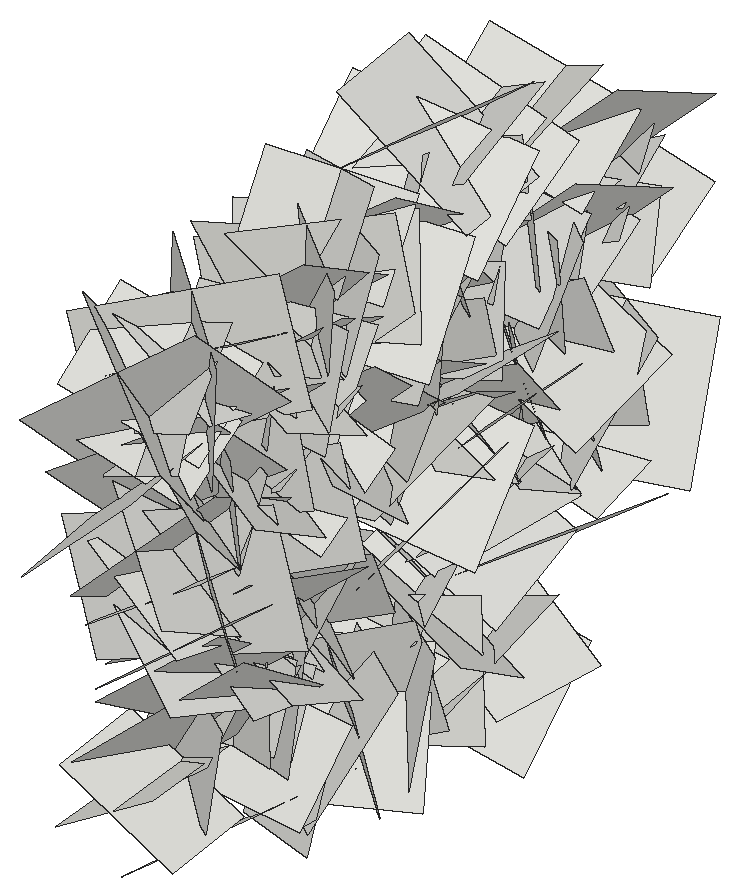
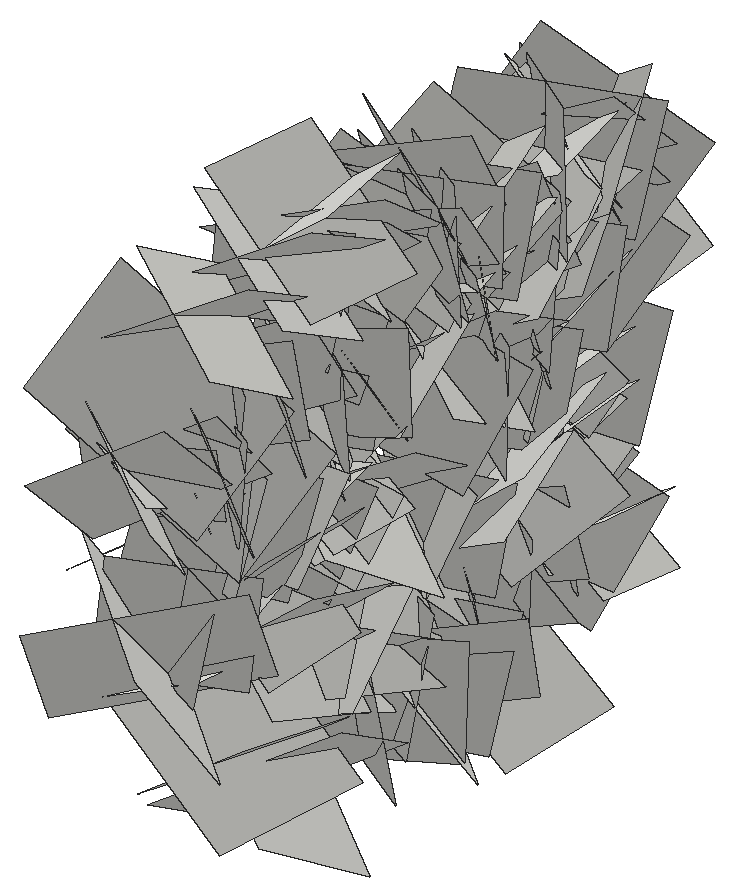
# SketchUp Ruby script. Lengths in inches.
U = 1.inch
M = Sketchup.active_model
def pt(a) = Geom::Point3d.new(a.map { |v| v * U })
def face(e, loops, mat)
  f = e.add_face(loops[0].map { |a| pt(a) })
  loops[1..].each { |l| e.add_face(l.map { |a| pt(a) }).erase! }
  f.material = f.back_material = mat if mat
  f
end
# faces: each face lists its corners as indices into pts; further lists are holes
def faces(e, pts, list, mat = nil) = list.each { |f| face(e, (f[0].is_a?(Array) ? f : [f]).map { |l| l.map { |i| pts[i] } }, mat) }
# xy, xz, yz: faces in a plane at the given z, y or x. An outline is a flat list of corners, or four numbers for a rectangle; further outlines are holes
def ring(l) = l.size == 4 ? [[l[0], l[1]], [l[2], l[1]], [l[2], l[3]], [l[0], l[3]]] : l.each_slice(2).to_a
def flat(e, list, mat, &to3) = list.each { |f| face(e, (f[0].is_a?(Array) ? f : [f]).map { |l| ring(l).map { |u, v| to3.(u, v) } }, mat) }
def xy(e, z, list, mat = nil) = flat(e, list, mat) { |x, y| [x, y, z] }
def xz(e, y, list, mat = nil) = flat(e, list, mat) { |x, z| [x, y, z] }
def yz(e, x, list, mat = nil) = flat(e, list, mat) { |y, z| [x, y, z] }
def lines(e, pts, list) = list.each { |a, b| e.add_line(pt(pts[a]), pt(pts[b])) }
# prism: a flat outline (further loops are holes) pulled along v
def prism(e, loops, v, mat = nil)
  f = face(e, loops, mat); d = Geom::Vector3d.new(v.map { |x| x * U })
  f.pushpull(f.normal.samedirection?(d) ? d.length : -d.length)
end
def box(e, o, s, mat = nil) = prism(e, [[o, [o[0] + s[0], o[1], o[2]], [o[0] + s[0], o[1] + s[1], o[2]], [o[0], o[1] + s[1], o[2]]]], [0, 0, s[2]], mat)
def at(x, y, z, deg = 0) = Geom::Transformation.translation(pt([x, y, z])) * Geom::Transformation.rotation(ORIGIN, Z_AXIS, deg.degrees)
def axes(o, x, y, z) = Geom::Transformation.new([*x, 0, *y, 0, *z, 0, *pt(o).to_a, 1])
def part(name) = M.definitions.add(name)
# library, detail: a bought-in or finely detailed component or shape, given as its bounding box
def library(name, o, s) = part(name).tap { |d| box(d.entities, o, s) }
def detail(e, o, s) = box(e.add_group.entities, o, s)
def put(e, d, t, mat = nil) = e.add_instance(d, t).tap { |i| i.material = mat if mat }
def group(e, t, mat = nil) = e.add_group.tap { |g| g.transformation = t; g.material = mat if mat }.entities
root = M.entities
c1 = part("Component\#6")
p = [[0.01,0,0],[0,3.24,4.54],[4.32,3.24,4.54],[4.33,0,0]]
faces(c1.entities,p,[[0,1,2,3]])
put(root,c1,axes([400.91,192.58,32.17],[0.11188,-0.86522,-0.03173],[-0.14554,-0.04829,0.85998],[0.90613,0.09907,0.14204]))
put(root,c1,axes([400.91,194.3125,23.26],[-0.02367,-0.75059,-0.08188],[0.02978,-0.08269,0.75031],[0.79979,-0.01914,-0.03036]))
put(root,c1,axes([404.88,194.3125,23.26],[0.02367,-0.75059,-0.08188],[-0.02978,-0.08269,0.75031],[-0.79979,-0.01914,-0.03036]))
put(root,c1,axes([400.91,192.15,39.48],[-0.21361,0.71392,-0.72381],[-0.12034,-0.74908,-0.70723],[1.07091,0.05823,-0.22384]))
put(root,c1,axes([404.88,192.15,39.48],[0.21361,0.71392,-0.72381],[0.12034,-0.74908,-0.70723],[-1.07091,0.05823,-0.22384]))
put(root,c1,axes([404.88,191.375,35.34],[-0.1473,0.40574,0.51918],[-0.07991,0.51733,-0.42447],[-0.69387,-0.14571,-0.06134]))
put(root,c1,axes([400.91,191.375,35.34],[0.1473,0.40574,0.51918],[0.07991,0.51733,-0.42447],[0.69387,-0.14571,-0.06134]))
put(root,c1,axes([404.88,195.16,37.28],[-0.08536,-0.54597,-0.55526],[-0.06407,-0.55215,0.55168],[-0.82294,0.09962,0.01464]))
put(root,c1,axes([400.91,195.16,37.28],[0.08536,-0.54597,-0.55526],[0.06407,-0.55215,0.55168],[0.82294,0.09962,0.01464]))
put(root,c1,axes([400.91,194.17,31.15],[-0.1572,-0.65225,0.62778],[-0.00257,0.63643,0.66066],[0.9596,-0.10514,0.10461]))
put(root,c1,axes([404.88,194.17,31.15],[0.1572,-0.65225,0.62778],[0.00257,0.63643,0.66066],[-0.9596,-0.10514,0.10461]))
put(root,c1,axes([400.91,192.38,31.46],[0.05244,0.73173,-0.11131],[0.01157,-0.11227,-0.73318],[0.78447,-0.04726,0.01825]))
put(root,c1,axes([404.88,192.38,31.46],[-0.05244,0.73173,-0.11131],[-0.01157,-0.11227,-0.73318],[-0.78447,-0.04726,0.01825]))
put(root,c1,axes([400.91,192.76,27.5],[-0.21382,-0.08753,1.03604],[0.20559,1.03367,0.1251],[1.08277,-0.21355,0.18084]))
put(root,c1,axes([400.91,193.07,33.95],[0.05953,0.85388,-0.40475],[-0.24794,-0.38029,-0.83472],[0.97048,-0.14953,-0.18843]))
put(root,c1,axes([404.88,193.07,33.95],[-0.05953,0.85388,-0.40475],[0.24794,-0.38029,-0.83472],[-0.97048,-0.14953,-0.18843]))
put(root,c1,axes([404.88,192.62,23.41],[0.0945,0.05137,0.75973],[-0.00531,0.76494,-0.05113],[-0.80713,0.00098,0.08928]))
put(root,c1,axes([404.88,193.25,29.42],[0.0602,0.67546,-0.3863],[0.10598,-0.39045,-0.66802],[-0.81797,-0.00088,-0.11498]))
put(root,c1,axes([400.91,194.92,22.54],[0.07164,-0.895,0.57486],[-0.24411,0.55005,0.88344],[1.1008,0.18023,0.15849]))
put(root,c1,axes([404.88,192.68,25.51],[-0.10584,0.56729,0.32604],[0.07365,0.33715,-0.56532],[-0.68964,-0.05105,-0.11041]))
put(root,c1,axes([404.88,195.4,26.27],[-0.15303,-0.80886,0.21466],[0.08059,0.20425,0.82078],[-0.8834,0.15875,0.0377]))
put(root,c1,axes([400.91,195.4,26.27],[0.15303,-0.80886,0.21466],[-0.08059,0.20425,0.82078],[0.8834,0.15875,0.0377]))
put(root,c1,axes([400.91,192.92,34.17],[-0.15147,-0.1521,1.01718],[-0.1212,1.02293,0.1369],[1.08344,0.09316,0.15752]))
put(root,c1,axes([404.88,192.92,34.17],[0.15147,-0.1521,1.01718],[0.1212,1.02293,0.1369],[-1.08344,0.09316,0.15752]))
put(root,c1,axes([400.91,195.89,35.57],[-0.03273,-0.74668,0.19464],[0.06894,0.19158,0.74527],[0.81502,-0.04619,-0.05522]))
put(root,c1,axes([404.88,195.89,35.57],[0.03273,-0.74668,0.19464],[-0.06894,0.19158,0.74527],[-0.81502,-0.04619,-0.05522]))
put(root,c1,axes([404.88,194.0625,27.88],[0.03826,-0.32146,0.75655],[0.14724,0.74878,0.31153],[-0.85881,0.11405,0.08712]))
put(root,c1,axes([404.88,194.18,31.13],[0.04063,-0.16003,0.87853],[0.02386,0.87924,0.15917],[-0.94627,0.0153,0.04174]))
put(root,c1,axes([400.91,194.18,31.13],[-0.04063,-0.16003,0.87853],[-0.02386,0.87924,0.15917],[0.94627,0.0153,0.04174]))
put(root,c1,axes([404.88,194.1,30.97],[0.07757,0.18705,0.69229],[-0.05179,0.69557,-0.18277],[-0.75837,-0.02837,0.08329]))
put(root,c1,axes([400.91,194.12,36.42],[-0.16155,0.92195,-0.51802],[0.06641,-0.51458,-0.93426],[1.119,0.16364,-0.01934]))
put(root,c1,axes([404.88,194.71,36.49],[0.01491,0.71707,-0.22931],[0.11795,-0.22881,-0.70868],[-0.78925,-0.02064,-0.11024]))
put(root,c1,axes([404.88,197.53,26.62],[-0.11622,-0.11144,-0.6986],[-0.08861,-0.69994,0.12478],[-0.74462,0.10068,0.09418]))
put(root,c1,axes([400.91,197.53,26.62],[0.11622,-0.11144,-0.6986],[0.08861,-0.69994,0.12478],[0.74462,0.10068,0.09418]))
put(root,c1,axes([404.88,198.41,25.5],[0.14641,-1.02966,0.26735],[0.10928,0.28128,1.03005],[-1.12233,-0.10694,0.13517]))
put(root,c1,axes([400.91,198.41,25.5],[-0.14641,-1.02966,0.26735],[-0.10928,0.28128,1.03005],[1.12233,-0.10694,0.13517]))
put(root,c1,axes([400.91,198.72,19.65],[-0.06387,-1.04135,0.05905],[-0.06023,0.06234,1.04135],[1.10396,-0.05685,0.06023]))
put(root,c1,axes([400.91,195.45,23.05],[0.08121,0.42866,0.62692],[0.16296,0.6083,-0.43472],[0.78836,-0.1699,0.02528]))
put(root,c1,axes([400.91,198.57,33.25],[-0.09717,0.14422,-0.89801],[-0.11089,-0.89824,-0.13357],[0.95769,-0.08937,-0.10658]))
put(root,c1,axes([404.88,198.57,33.25],[0.09717,0.14422,-0.89801],[0.11089,-0.89824,-0.13357],[-0.95769,-0.08937,-0.10658]))
put(root,c1,axes([400.91,195.7,29.31],[-0.12944,0.87645,-0.3909],[0.13192,-0.37627,-0.88251],[1.00866,0.16168,0.06525]))
put(root,c1,axes([400.91,196.41,37.05],[0.02372,0.78814,-0.36288],[0.15491,-0.36124,-0.77556],[0.90659,0.0411,0.14202]))
put(root,c1,axes([404.88,195.33,34.42],[-0.12228,0.30682,0.85432],[0.19875,0.85067,-0.2802],[-0.94146,0.13973,-0.17012]))
put(root,c1,axes([400.91,195.33,34.42],[0.12228,0.30682,0.85432],[-0.19875,0.85067,-0.2802],[0.94146,0.13973,-0.17012]))
put(root,c1,axes([400.91,200.17,25.9],[0.12286,-0.34825,-0.84521],[-0.12526,-0.85054,0.33424],[0.96086,-0.06635,0.15165]))
put(root,c1,axes([400.91,196.95,39.61],[-0.06663,0.78722,-0.39485],[-0.0883,-0.3994,-0.78302],[0.92935,0.01849,-0.10271]))
put(root,c1,axes([404.88,196.95,39.61],[0.06663,0.78722,-0.39485],[0.0883,-0.3994,-0.78302],[-0.92935,0.01849,-0.10271]))
put(root,c1,axes([404.88,199.74,34.07],[-0.11183,-0.60219,-0.2199],[0.02555,-0.22643,0.6085],[-0.67907,0.09065,0.0591]))
put(root,c1,axes([404.88,197.11,20.7],[0.0234,0.20043,0.60552],[-0.11848,0.59772,-0.19378],[-0.66563,-0.09934,0.05578]))
put(root,c1,axes([404.88,201.02,32],[0.03236,-0.79816,-0.43551],[0.07074,-0.43262,0.79753],[-0.9612,-0.0587,0.04403]))
put(root,c1,axes([400.91,201.02,32],[-0.03236,-0.79816,-0.43551],[-0.07074,-0.43262,0.79753],[0.9612,-0.0587,0.04403]))
put(root,c1,axes([400.91,200.08,36.17],[0.04967,-0.3024,-0.77978],[0.15753,-0.76557,0.30582],[0.87244,0.15545,-0.01082]))
put(root,c1,axes([404.88,196.5,26.6],[0.00001,0.64808,0.59207],[0.20568,0.57742,-0.63205],[-0.90746,0.13088,-0.14325]))
put(root,c1,axes([404.88,198.68,37.125],[-0.06347,0.58127,-0.24952],[0.07215,-0.24326,-0.58302],[-0.66662,-0.08167,-0.03935]))
put(root,c1,axes([400.91,201.02,39.48],[-0.13577,0.09163,-0.9618],[-0.05798,-0.96935,-0.08506],[1.02248,-0.0428,-0.13253]))
put(root,c1,axes([404.88,201.02,39.48],[0.13577,0.09163,-0.9618],[0.05798,-0.96935,-0.08506],[-1.02248,-0.0428,-0.13253]))
put(root,c1,axes([404.88,199.18,25.47],[-0.11604,-0.3767,0.6399],[0.02749,0.64448,0.38383],[-0.78661,0.07809,-0.08099]))
put(root,c1,axes([400.91,199.18,25.47],[0.11604,-0.3767,0.6399],[-0.02749,0.64448,0.38383],[0.78661,0.07809,-0.08099]))
put(root,c1,axes([400.91,197.17,21.41],[-0.31691,0.51794,0.91951],[-0.05422,0.94746,-0.55031],[1.11735,0.19287,0.23409]))
put(root,c1,axes([404.88,197.17,21.41],[0.31691,0.51794,0.91951],[0.05422,0.94746,-0.55031],[-1.11735,0.19287,0.23409]))
put(root,c1,axes([400.91,202.06,39.63],[-0.00244,-0.36914,-0.6705],[0.07457,-0.66776,0.36739],[0.80789,0.06052,-0.03594]))
put(root,c1,axes([404.88,202.06,39.63],[0.00244,-0.36914,-0.6705],[-0.07457,-0.66776,0.36739],[-0.80789,0.06052,-0.03594]))
put(root,c1,axes([404.88,198.86,35.2],[0.14047,0.16017,0.87964],[-0.13868,0.88315,-0.1411],[-0.93754,-0.10664,0.15267]))
put(root,c1,axes([400.91,198.86,35.2],[-0.14047,0.16017,0.87964],[0.13868,0.88315,-0.1411],[0.93754,-0.10664,0.15267]))
put(root,c1,axes([404.88,200.1,34.99],[-0.01875,0.74709,-0.59948],[0.09315,-0.59579,-0.74508],[-1.01106,-0.06874,-0.05753]))
put(root,c1,axes([400.91,200.1,34.99],[0.01875,0.74709,-0.59948],[-0.09315,-0.59579,-0.74508],[1.01106,-0.06874,-0.05753]))
put(root,c1,axes([404.88,201.91,26.14],[0.02369,0.31708,-0.9382],[0.09459,-0.93526,-0.31396],[-1.04548,-0.07743,-0.04967]))
put(root,c1,axes([400.91,201.91,26.14],[-0.02369,0.31708,-0.9382],[-0.09459,-0.93526,-0.31396],[1.04548,-0.07743,-0.04967]))
put(root,c1,axes([400.91,198.67,35.61],[-0.10111,0.59855,0.78971],[0.15679,0.79307,-0.58323],[1.03859,-0.06146,0.16492]))
put(root,c1,axes([404.88,201.07,39.9375],[0.03161,0.68058,-0.41337],[0.06223,-0.41441,-0.67806],[-0.84176,-0.00508,-0.06565]))
put(root,c1,axes([400.91,206.72,25.52],[-0.07134,-1.27871,-0.42932],[-0.37284,-0.39835,1.24159],[1.38032,-0.17369,0.31318]))
put(root,c1,axes([404.88,204.82,25.65],[0.12938,-0.11687,-1.00907],[-0.02351,-1.01639,0.11504],[-1.07651,0.00815,-0.12379]))
put(root,c1,axes([400.91,204.82,25.65],[-0.12938,-0.11687,-1.00907],[0.02351,-1.01639,0.11504],[1.07651,0.00815,-0.12379]))
put(root,c1,axes([400.91,204.74,34.65],[0.08046,-0.48471,-0.63269],[0.12911,-0.62103,0.49039],[0.83492,0.14274,-0.01486]))
put(root,c1,axes([404.88,200.85,29.625],[0.04324,0.39016,0.69087],[0.10275,0.68414,-0.39209],[-0.83473,0.10443,-0.01247]))
put(root,c1,axes([404.88,202.42,34.22],[0.03507,0.56649,-0.26791],[-0.06705,-0.26389,-0.56581],[-0.66085,0.05684,0.04319]))
put(root,c1,axes([400.91,205,37.54],[0.1597,-0.46751,-0.41946],[-0.05532,-0.43919,0.47075],[0.66349,0.07592,0.14021]))
put(root,c1,axes([404.88,205,37.54],[-0.1597,-0.46751,-0.41946],[0.05532,-0.43919,0.47075],[-0.66349,0.07592,0.14021]))
put(root,c1,axes([400.91,201.89,25.36],[0.12511,0.60489,0.30184],[-0.04372,0.31228,-0.60968],[0.71524,-0.08672,-0.09007]))
put(root,c1,axes([404.88,201.89,25.36],[-0.12511,0.60489,0.30184],[0.04372,0.31228,-0.60968],[-0.71524,-0.08672,-0.09007]))
put(root,c1,axes([404.88,200.125,30.08],[0.25415,0.9144,0.59243],[0.00684,0.60541,-0.93704],[-1.1549,0.20481,0.12483]))
put(root,c1,axes([400.91,200.125,30.08],[-0.25415,0.9144,0.59243],[-0.00684,0.60541,-0.93704],[1.1549,0.20481,0.12483]))
put(root,c1,axes([400.91,201.41,38.375],[-0.12316,0.77538,0.57304],[0.12545,0.58429,-0.76661],[1.01427,0.02189,0.1644]))
put(root,c1,axes([404.88,204.22,36.67],[-0.08595,0.41822,-0.43473],[0.01861,-0.43682,-0.42351],[-0.63917,-0.06896,0.04613]))
put(root,c1,axes([404.88,204.95,35.05],[-0.03568,0.1968,-0.61743],[0.04358,-0.61637,-0.1987],[-0.68554,-0.04943,0.01951]))
put(root,c1,axes([400.91,202.75,27.49],[-0.17368,0.85862,-0.51485],[0.1903,-0.48804,-0.87105],[1.04401,0.2318,0.07312]))
put(root,c1,axes([400.91,202.89,32.22],[-0.0211,0.0618,0.84202],[-0.01452,0.84212,-0.06213],[0.89482,0.01512,0.01885]))
put(root,c1,axes([404.88,202.89,32.22],[0.0211,0.0618,0.84202],[0.01452,0.84212,-0.06213],[-0.89482,0.01512,0.01885]))
put(root,c1,axes([404.88,202.23,33.91],[-0.02493,0.60398,0.49928],[0.17768,0.49182,-0.58706],[-0.81142,0.08914,-0.14389]))
put(root,c1,axes([404.88,204.33,34.72],[0.02793,-0.28222,0.66343],[-0.05268,0.66158,0.28341],[-0.7624,-0.05605,0.00473]))
put(root,c1,axes([400.91,207.21,30.03],[-0.00943,-1.01637,-0.0193],[-0.00822,-0.01923,1.01638],[1.07752,-0.00904,0.00758]))
put(root,c1,axes([400.91,207.4,37.82],[-0.14382,-0.92009,0.02073],[-0.06912,0.03051,0.92748],[0.97309,-0.13382,0.06894]))
put(root,c1,axes([404.88,207.4,37.82],[0.14382,-0.92009,0.02073],[0.06912,0.03051,0.92748],[-0.97309,-0.13382,0.06894]))
put(root,c1,axes([404.88,204.65,32.19],[-0.14144,0.68446,-0.34907],[-0.03425,-0.35898,-0.69154],[-0.81371,-0.10387,0.08978]))
put(root,c1,axes([400.91,204.65,32.19],[0.14144,0.68446,-0.34907],[0.03425,-0.35898,-0.69154],[0.81371,-0.10387,0.08978]))
put(root,c1,axes([404.88,206.625,39.5],[0.00312,0.09172,-0.66161],[-0.00201,-0.66161,-0.09173],[-0.70801,0.00228,-0.00265]))
put(root,c1,axes([404.88,206.58,28.49],[-0.01093,-0.51913,0.63451],[-0.10311,0.63085,0.51456],[-0.86287,-0.06881,-0.06953]))
put(root,c1,axes([400.91,206.58,28.49],[0.01093,-0.51913,0.63451],[0.10311,0.63085,0.51456],[0.86287,-0.06881,-0.06953]))
put(root,c1,axes([404.88,209.1,25.86],[0.06992,-0.92649,-0.30548],[0.11921,-0.29692,0.92479],[-1.02719,-0.09753,0.08653]))
put(root,c1,axes([400.91,209.1,25.86],[-0.06992,-0.92649,-0.30548],[-0.11921,-0.29692,0.92479],[1.02719,-0.09753,0.08653]))
put(root,c1,axes([404.88,209.72,22.08],[0.18138,-0.91546,-0.54155],[0.07402,-0.53767,0.93095],[-1.12504,-0.18297,-0.02606]))
put(root,c1,axes([400.91,209.72,22.08],[-0.18138,-0.91546,-0.54155],[-0.07402,-0.53767,0.93095],[1.12504,-0.18297,-0.02606]))
put(root,c1,axes([404.88,204.07,39.0625],[0.02986,0.79051,0.40956],[-0.00815,0.40997,-0.79076],[-0.94369,0.02147,0.01979]))
put(root,c1,axes([400.91,204.07,39.0625],[-0.02986,0.79051,0.40956],[0.00815,0.40997,-0.79076],[0.94369,0.02147,0.01979]))
put(root,c1,axes([404.88,209.27,26.87],[-0.02942,-0.98917,0.00062],[0.2303,-0.00549,0.9654],[-1.02292,0.02721,0.21733]))
put(root,c1,axes([400.91,209.27,26.87],[0.02942,-0.98917,0.00062],[-0.2303,-0.00549,0.9654],[1.02292,0.02721,0.21733]))
put(root,c1,axes([404.88,205.35,34.65],[-0.12302,0.37909,0.72016],[0.00858,0.72795,-0.38188],[-0.86263,-0.04682,-0.1065]))
put(root,c1,axes([400.91,205.35,34.65],[0.12302,0.37909,0.72016],[-0.00858,0.72795,-0.38188],[0.86263,-0.04682,-0.1065]))
put(root,c1,axes([400.91,205.67,24.52],[0.15369,0.87531,0.08009],[-0.01982,0.08422,-0.88666],[0.9315,-0.14262,-0.03208]))
put(root,c1,axes([404.88,206.77,29.69],[-0.13468,0.0618,0.68245],[0.14259,0.68282,-0.03679],[-0.71222,0.12502,-0.13642]))
put(root,c1,axes([404.88,209.27,26.93],[-0.01951,-0.6006,0.29742],[-0.06663,0.29777,0.59742],[-0.70729,-0.01148,-0.06448]))
put(root,c1,axes([400.91,211.47,22.62],[-0.20513,-1.22241,0.07319],[-0.04122,0.08019,1.23659],[1.29742,-0.19072,0.05085]))
put(root,c1,axes([400.91,209.37,33.75],[-0.00852,0.3462,-0.76666],[-0.09329,-0.76284,-0.34355],[0.88678,-0.07692,-0.04351]))
put(root,c1,axes([404.88,209.37,33.75],[0.00852,0.3462,-0.76666],[0.09329,-0.76284,-0.34355],[-0.88678,-0.07692,-0.04351]))
put(root,c1,axes([400.91,207.43,34.16],[0.11276,0.04323,0.70746],[-0.03845,0.71477,-0.03823],[0.75032,0.03013,-0.10828]))
put(root,c1,axes([404.88,207.43,34.16],[-0.11276,0.04323,0.70746],[0.03845,0.71477,-0.03823],[-0.75032,0.03013,-0.10828]))
put(root,c1,axes([400.91,210.23,35.31],[0.06568,0.00099,-0.81141],[0.08224,-0.81005,0.00494],[0.85616,0.07773,0.06177]))
put(root,c1,axes([400.91,206.36,33.23],[-0.09168,1.1059,0.20164],[-0.04784,0.19866,-1.1089],[1.19063,0.09314,-0.02903]))
put(root,c1,axes([404.88,207.11,31.75],[0.23783,0.22127,0.93353],[0.03566,0.95632,-0.23476],[-1.01634,0.08533,0.21022]))
put(root,c1,axes([400.91,210.61,30.96],[0.02538,-1.03384,0.49264],[-0.2847,0.47394,1.00764],[1.18007,0.13657,0.23251]))
put(root,c1,axes([400.91,211.91,37.97],[-0.10192,-0.72839,-0.40458],[-0.00784,-0.4065,0.73361],[0.88316,-0.08767,-0.04018]))
put(root,c1,axes([404.88,211.91,37.97],[0.10192,-0.72839,-0.40458],[0.00784,-0.4065,0.73361],[-0.88316,-0.08767,-0.04018]))
put(root,c1,axes([400.91,209.14,33.82],[0.16184,0.36707,0.52708],[-0.01835,0.54392,-0.37378],[0.68059,-0.07262,-0.13541]))
put(root,c1,axes([404.88,209.14,33.82],[-0.16184,0.36707,0.52708],[0.01835,0.54392,-0.37378],[-0.68059,-0.07262,-0.13541]))
put(root,c1,axes([404.88,212.36,26.625],[0.06935,-0.64087,-0.11796],[-0.11905,-0.12787,0.63241],[-0.68039,-0.04294,-0.12268]))
put(root,c1,axes([404.88,210.17,27.25],[-0.0389,-0.19659,0.74237],[-0.03773,0.74285,0.19496],[-0.81316,-0.02506,-0.04456]))
put(root,c1,axes([400.91,210.17,27.25],[0.0389,-0.19659,0.74237],[0.03773,0.74285,0.19496],[0.81316,-0.02506,-0.04456]))
put(root,c1,axes([400.91,212.48,33.12],[0.02538,-1.03384,0.49264],[-0.2847,0.47394,1.00764],[1.18007,0.13657,0.23251]))
put(root,c1,axes([404.88,212.78,35.18],[0.06835,-0.19577,-0.64021],[-0.13077,-0.63563,0.18195],[-0.69749,0.09999,-0.09685]))
put(root,c1,axes([404.88,208.86,27.22],[0.22907,0.58895,0.94038],[0.09031,0.94642,-0.61231],[-1.17269,0.18793,0.13653]))
put(root,c1,axes([400.91,208.86,27.22],[-0.22907,0.58895,0.94038],[-0.09031,0.94642,-0.61231],[1.17269,0.18793,0.13653]))
put(root,c1,axes([404.88,211.1,35.2],[-0.07899,0.5337,0.27791],[-0.02897,0.27674,-0.53878],[-0.63716,-0.07875,-0.00996]))
put(root,c1,axes([404.88,210.92,34.25],[-0.13403,0.53039,0.57824],[0.04314,0.58935,-0.53168],[-0.83061,-0.05497,-0.12092]))
put(root,c1,axes([400.91,210.92,34.25],[0.13403,0.53039,0.57824],[-0.04314,0.58935,-0.53168],[0.83061,-0.05497,-0.12092]))
